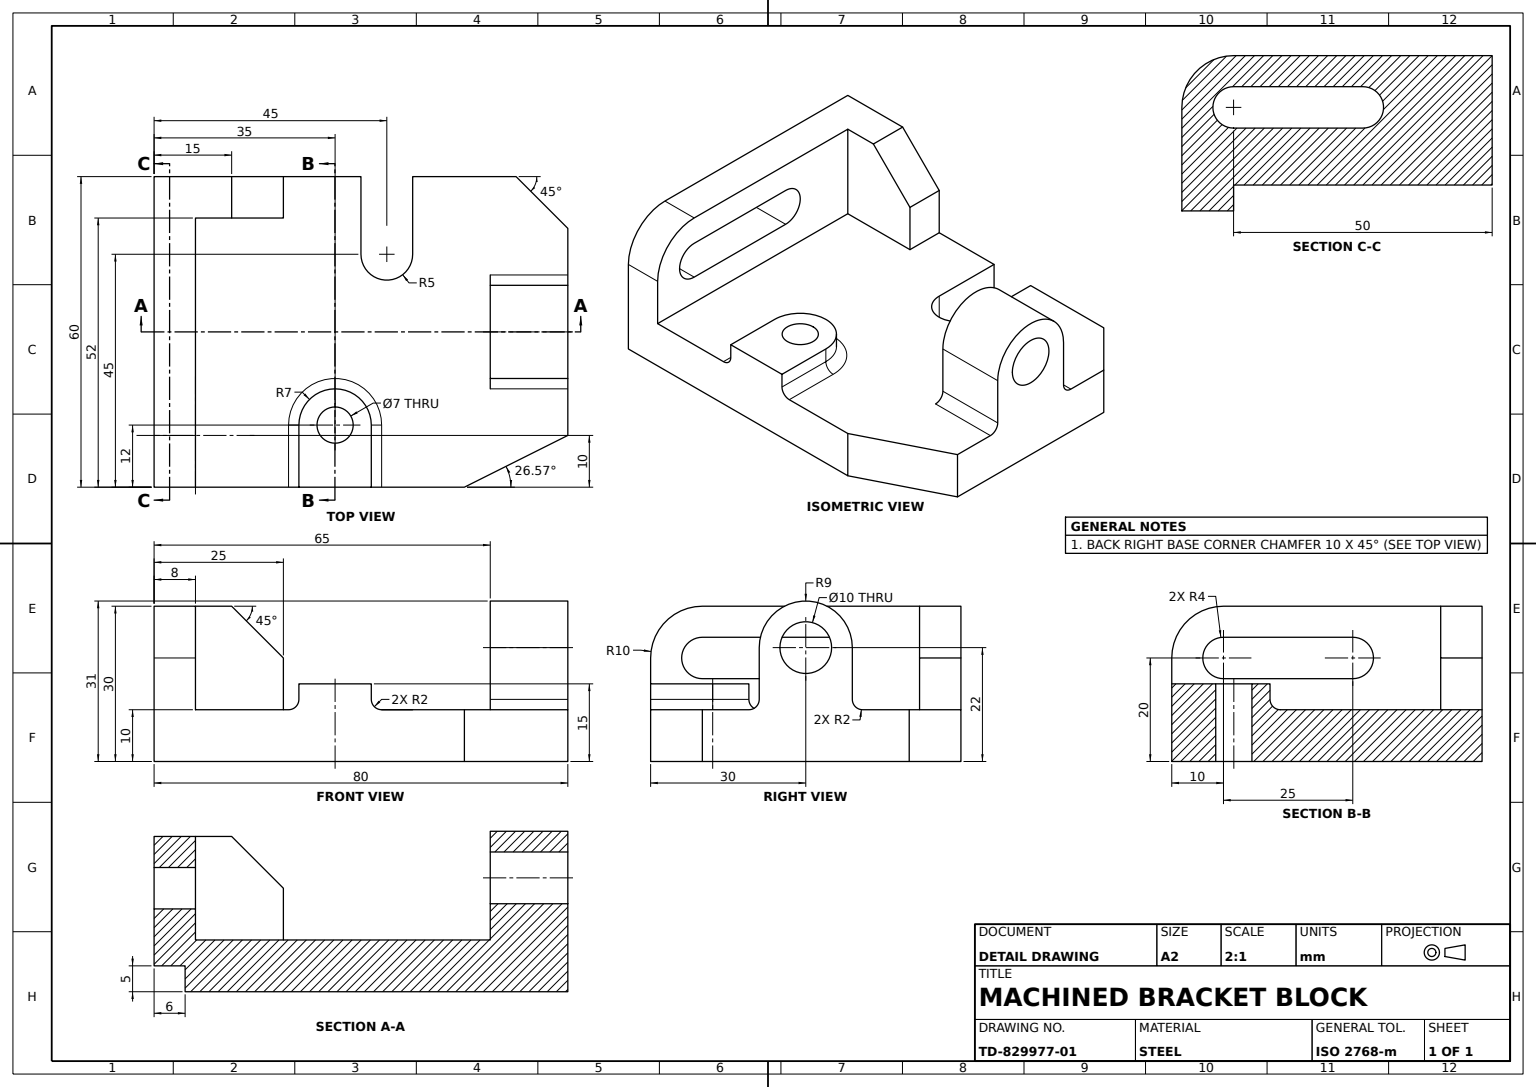
ISO-10303-21;
HEADER;
FILE_DESCRIPTION((''),'2;1');
FILE_NAME('','',(''),(''),'','','');
FILE_SCHEMA(('AUTOMOTIVE_DESIGN'));
ENDSEC;
DATA;
#1=APPLICATION_CONTEXT('');
#2=PRODUCT_CONTEXT('',#1,'mechanical');
#3=PRODUCT('','','',(#2));
#4=PRODUCT_DEFINITION_FORMATION('','',#3);
#5=PRODUCT_DEFINITION_CONTEXT('',#1,'design');
#6=PRODUCT_DEFINITION('','',#4,#5);
#7=PRODUCT_DEFINITION_SHAPE('','',#6);
#8=(LENGTH_UNIT()NAMED_UNIT(*)SI_UNIT(.MILLI.,.METRE.));
#9=(NAMED_UNIT(*)PLANE_ANGLE_UNIT()SI_UNIT($,.RADIAN.));
#10=(NAMED_UNIT(*)SI_UNIT($,.STERADIAN.)SOLID_ANGLE_UNIT());
#11=UNCERTAINTY_MEASURE_WITH_UNIT(LENGTH_MEASURE(1.E-05),#8,'distance_accuracy_value','');
#12=(GEOMETRIC_REPRESENTATION_CONTEXT(3)GLOBAL_UNCERTAINTY_ASSIGNED_CONTEXT((#11))GLOBAL_UNIT_ASSIGNED_CONTEXT((#8,#9,#10))REPRESENTATION_CONTEXT('',''));
#13=CARTESIAN_POINT('',(42.,15.,30.));
#14=VERTEX_POINT('',#13);
#15=CARTESIAN_POINT('',(42.,12.,30.));
#16=VERTEX_POINT('',#15);
#17=DIRECTION('',(0.,-1.,0.));
#18=VECTOR('',#17,1000.);
#19=LINE('',#13,#18);
#20=EDGE_CURVE('',#14,#16,#19,.T.);
#21=ORIENTED_EDGE('',*,*,#20,.T.);
#22=CARTESIAN_POINT('',(42.,12.,18.));
#23=VERTEX_POINT('',#22);
#24=DIRECTION('',(0.,0.,-1.));
#25=VECTOR('',#24,1000.);
#26=LINE('',#15,#25);
#27=EDGE_CURVE('',#16,#23,#26,.T.);
#28=ORIENTED_EDGE('',*,*,#27,.T.);
#29=CARTESIAN_POINT('',(42.,15.,18.));
#30=VERTEX_POINT('',#29);
#31=LINE('',#29,#18);
#32=EDGE_CURVE('',#30,#23,#31,.T.);
#33=ORIENTED_EDGE('',*,*,#32,.F.);
#34=LINE('',#13,#25);
#35=EDGE_CURVE('',#14,#30,#34,.T.);
#36=ORIENTED_EDGE('',*,*,#35,.F.);
#37=EDGE_LOOP('',(#21,#28,#33,#36));
#38=FACE_OUTER_BOUND('',#37,.T.);
#39=DIRECTION('',(-1.,0.,0.));
#40=DIRECTION('',(0.,0.,1.));
#41=AXIS2_PLACEMENT_3D('',#13,#39,#40);
#42=PLANE('',#41);
#43=ADVANCED_FACE('',(#38),#42,.F.);
#44=CARTESIAN_POINT('',(28.,15.,18.));
#45=VERTEX_POINT('',#44);
#46=CARTESIAN_POINT('',(28.,12.,18.));
#47=VERTEX_POINT('',#46);
#48=LINE('',#44,#18);
#49=EDGE_CURVE('',#45,#47,#48,.T.);
#50=ORIENTED_EDGE('',*,*,#49,.F.);
#51=CARTESIAN_POINT('',(35.,15.,11.));
#52=VERTEX_POINT('',#51);
#53=CARTESIAN_POINT('',(35.,15.,18.));
#54=DIRECTION('',(0.,1.,0.));
#55=AXIS2_PLACEMENT_3D('',#53,#54,#40);
#56=CIRCLE('',#55,7.);
#57=EDGE_CURVE('',#52,#45,#56,.T.);
#58=ORIENTED_EDGE('',*,*,#57,.F.);
#59=CARTESIAN_POINT('',(35.,12.,11.));
#60=VERTEX_POINT('',#59);
#61=LINE('',#51,#18);
#62=EDGE_CURVE('',#52,#60,#61,.T.);
#63=ORIENTED_EDGE('',*,*,#62,.T.);
#64=CARTESIAN_POINT('',(35.,12.,18.));
#65=AXIS2_PLACEMENT_3D('',#64,#54,#40);
#66=CIRCLE('',#65,7.);
#67=EDGE_CURVE('',#60,#47,#66,.T.);
#68=ORIENTED_EDGE('',*,*,#67,.T.);
#69=EDGE_LOOP('',(#50,#58,#63,#68));
#70=FACE_OUTER_BOUND('',#69,.T.);
#71=AXIS2_PLACEMENT_3D('',#53,#17,#24);
#72=CYLINDRICAL_SURFACE('',#71,7.);
#73=ADVANCED_FACE('',(#70),#72,.T.);
#74=CARTESIAN_POINT('',(0.,20.,24.));
#75=VERTEX_POINT('',#74);
#76=CARTESIAN_POINT('',(0.,24.,20.));
#77=VERTEX_POINT('',#76);
#78=CARTESIAN_POINT('',(0.,20.,20.));
#79=AXIS2_PLACEMENT_3D('',#78,#39,#40);
#80=CIRCLE('',#79,4.);
#81=EDGE_CURVE('',#75,#77,#80,.T.);
#82=ORIENTED_EDGE('',*,*,#81,.T.);
#83=CARTESIAN_POINT('',(8.,24.,20.));
#84=VERTEX_POINT('',#83);
#85=VECTOR('',#39,1000.);
#86=LINE('',#83,#85);
#87=EDGE_CURVE('',#84,#77,#86,.T.);
#88=ORIENTED_EDGE('',*,*,#87,.F.);
#89=CARTESIAN_POINT('',(8.,20.,24.));
#90=VERTEX_POINT('',#89);
#91=CARTESIAN_POINT('',(8.,20.,20.));
#92=AXIS2_PLACEMENT_3D('',#91,#39,#40);
#93=CIRCLE('',#92,4.);
#94=EDGE_CURVE('',#90,#84,#93,.T.);
#95=ORIENTED_EDGE('',*,*,#94,.F.);
#96=LINE('',#89,#85);
#97=EDGE_CURVE('',#90,#75,#96,.T.);
#98=ORIENTED_EDGE('',*,*,#97,.T.);
#99=EDGE_LOOP('',(#82,#88,#95,#98));
#100=FACE_OUTER_BOUND('',#99,.T.);
#101=CYLINDRICAL_SURFACE('',#92,4.);
#102=ADVANCED_FACE('',(#100),#101,.F.);
#103=CARTESIAN_POINT('',(0.,16.,-5.));
#104=VERTEX_POINT('',#103);
#105=CARTESIAN_POINT('',(0.,16.,20.));
#106=VERTEX_POINT('',#105);
#107=VECTOR('',#40,1000.);
#108=LINE('',#105,#107);
#109=EDGE_CURVE('',#104,#106,#108,.T.);
#110=ORIENTED_EDGE('',*,*,#109,.F.);
#111=CARTESIAN_POINT('',(0.,24.,-5.));
#112=VERTEX_POINT('',#111);
#113=CARTESIAN_POINT('',(0.,20.,-5.));
#114=AXIS2_PLACEMENT_3D('',#113,#39,#40);
#115=CIRCLE('',#114,4.);
#116=EDGE_CURVE('',#112,#104,#115,.T.);
#117=ORIENTED_EDGE('',*,*,#116,.F.);
#118=LINE('',#76,#25);
#119=EDGE_CURVE('',#77,#112,#118,.T.);
#120=ORIENTED_EDGE('',*,*,#119,.F.);
#121=ORIENTED_EDGE('',*,*,#81,.F.);
#122=EDGE_CURVE('',#106,#75,#80,.T.);
#123=ORIENTED_EDGE('',*,*,#122,.F.);
#124=EDGE_LOOP('',(#110,#117,#120,#121,#123));
#125=FACE_BOUND('',#124,.T.);
#126=CARTESIAN_POINT('',(0.,0.,20.));
#127=VERTEX_POINT('',#126);
#128=CARTESIAN_POINT('',(0.,0.,30.));
#129=VERTEX_POINT('',#128);
#130=CARTESIAN_POINT('',(0.,0.,0.));
#131=LINE('',#130,#107);
#132=EDGE_CURVE('',#127,#129,#131,.T.);
#133=ORIENTED_EDGE('',*,*,#132,.T.);
#134=CARTESIAN_POINT('',(0.,20.,30.));
#135=VERTEX_POINT('',#134);
#136=CARTESIAN_POINT('',(0.,10.,30.));
#137=LINE('',#136,#18);
#138=EDGE_CURVE('',#135,#129,#137,.T.);
#139=ORIENTED_EDGE('',*,*,#138,.F.);
#140=CARTESIAN_POINT('',(0.,30.,20.));
#141=VERTEX_POINT('',#140);
#142=CIRCLE('',#79,10.);
#143=EDGE_CURVE('',#135,#141,#142,.T.);
#144=ORIENTED_EDGE('',*,*,#143,.T.);
#145=CARTESIAN_POINT('',(0.,30.,-30.));
#146=VERTEX_POINT('',#145);
#147=LINE('',#140,#25);
#148=EDGE_CURVE('',#141,#146,#147,.T.);
#149=ORIENTED_EDGE('',*,*,#148,.T.);
#150=CARTESIAN_POINT('',(0.,5.,-30.));
#151=VERTEX_POINT('',#150);
#152=CARTESIAN_POINT('',(0.,10.,-30.));
#153=LINE('',#152,#18);
#154=EDGE_CURVE('',#146,#151,#153,.T.);
#155=ORIENTED_EDGE('',*,*,#154,.T.);
#156=CARTESIAN_POINT('',(0.,5.,20.));
#157=VERTEX_POINT('',#156);
#158=LINE('',#156,#25);
#159=EDGE_CURVE('',#157,#151,#158,.T.);
#160=ORIENTED_EDGE('',*,*,#159,.F.);
#161=VECTOR('',#54,1000.);
#162=LINE('',#126,#161);
#163=EDGE_CURVE('',#127,#157,#162,.T.);
#164=ORIENTED_EDGE('',*,*,#163,.F.);
#165=EDGE_LOOP('',(#133,#139,#144,#149,#155,#160,#164));
#166=FACE_OUTER_BOUND('',#165,.T.);
#167=CARTESIAN_POINT('',(0.,10.,0.));
#168=DIRECTION('',(1.,0.,0.));
#169=AXIS2_PLACEMENT_3D('',#167,#168,#24);
#170=PLANE('',#169);
#171=ADVANCED_FACE('',(#125,#166),#170,.F.);
#172=CARTESIAN_POINT('',(8.,16.,-5.));
#173=VERTEX_POINT('',#172);
#174=CARTESIAN_POINT('',(8.,16.,20.));
#175=VERTEX_POINT('',#174);
#176=LINE('',#174,#107);
#177=EDGE_CURVE('',#173,#175,#176,.T.);
#178=ORIENTED_EDGE('',*,*,#177,.F.);
#179=LINE('',#172,#85);
#180=EDGE_CURVE('',#173,#104,#179,.T.);
#181=ORIENTED_EDGE('',*,*,#180,.T.);
#182=ORIENTED_EDGE('',*,*,#109,.T.);
#183=LINE('',#174,#85);
#184=EDGE_CURVE('',#175,#106,#183,.T.);
#185=ORIENTED_EDGE('',*,*,#184,.F.);
#186=EDGE_LOOP('',(#178,#181,#182,#185));
#187=FACE_OUTER_BOUND('',#186,.T.);
#188=AXIS2_PLACEMENT_3D('',#174,#17,#24);
#189=PLANE('',#188);
#190=ADVANCED_FACE('',(#187),#189,.F.);
#191=CARTESIAN_POINT('',(60.,10.,30.));
#192=VERTEX_POINT('',#191);
#193=CARTESIAN_POINT('',(80.,10.,20.));
#194=VERTEX_POINT('',#193);
#195=DIRECTION('',(0.894427191,0.,-0.447213595));
#196=VECTOR('',#195,1000.);
#197=LINE('',#193,#196);
#198=EDGE_CURVE('',#192,#194,#197,.T.);
#199=ORIENTED_EDGE('',*,*,#198,.T.);
#200=CARTESIAN_POINT('',(80.,10.,11.));
#201=VERTEX_POINT('',#200);
#202=CARTESIAN_POINT('',(80.,10.,-30.));
#203=LINE('',#202,#25);
#204=EDGE_CURVE('',#194,#201,#203,.T.);
#205=ORIENTED_EDGE('',*,*,#204,.T.);
#206=CARTESIAN_POINT('',(65.,10.,11.));
#207=VERTEX_POINT('',#206);
#208=LINE('',#206,#85);
#209=EDGE_CURVE('',#201,#207,#208,.T.);
#210=ORIENTED_EDGE('',*,*,#209,.T.);
#211=CARTESIAN_POINT('',(65.,10.,-11.));
#212=VERTEX_POINT('',#211);
#213=CARTESIAN_POINT('',(65.,10.,9.));
#214=LINE('',#213,#25);
#215=EDGE_CURVE('',#207,#212,#214,.T.);
#216=ORIENTED_EDGE('',*,*,#215,.T.);
#217=CARTESIAN_POINT('',(80.,10.,-11.));
#218=VERTEX_POINT('',#217);
#219=VECTOR('',#168,1000.);
#220=LINE('',#217,#219);
#221=EDGE_CURVE('',#212,#218,#220,.T.);
#222=ORIENTED_EDGE('',*,*,#221,.T.);
#223=CARTESIAN_POINT('',(80.,10.,-20.));
#224=VERTEX_POINT('',#223);
#225=EDGE_CURVE('',#218,#224,#203,.T.);
#226=ORIENTED_EDGE('',*,*,#225,.T.);
#227=CARTESIAN_POINT('',(70.,10.,-30.));
#228=VERTEX_POINT('',#227);
#229=CARTESIAN_POINT('',(65.,10.,-35.));
#230=DIRECTION('',(-0.707106781,0.,-0.707106781));
#231=VECTOR('',#230,1000.);
#232=LINE('',#229,#231);
#233=EDGE_CURVE('',#224,#228,#232,.T.);
#234=ORIENTED_EDGE('',*,*,#233,.T.);
#235=CARTESIAN_POINT('',(50.,10.,-30.));
#236=VERTEX_POINT('',#235);
#237=LINE('',#235,#85);
#238=EDGE_CURVE('',#228,#236,#237,.T.);
#239=ORIENTED_EDGE('',*,*,#238,.T.);
#240=CARTESIAN_POINT('',(50.,10.,-15.));
#241=VERTEX_POINT('',#240);
#242=LINE('',#240,#107);
#243=EDGE_CURVE('',#236,#241,#242,.T.);
#244=ORIENTED_EDGE('',*,*,#243,.T.);
#245=CARTESIAN_POINT('',(40.,10.,-15.));
#246=VERTEX_POINT('',#245);
#247=CARTESIAN_POINT('',(45.,10.,-15.));
#248=AXIS2_PLACEMENT_3D('',#247,#17,#40);
#249=CIRCLE('',#248,5.);
#250=EDGE_CURVE('',#241,#246,#249,.T.);
#251=ORIENTED_EDGE('',*,*,#250,.T.);
#252=CARTESIAN_POINT('',(40.,10.,-30.));
#253=VERTEX_POINT('',#252);
#254=LINE('',#252,#25);
#255=EDGE_CURVE('',#246,#253,#254,.T.);
#256=ORIENTED_EDGE('',*,*,#255,.T.);
#257=CARTESIAN_POINT('',(25.,10.,-30.));
#258=VERTEX_POINT('',#257);
#259=LINE('',#152,#85);
#260=EDGE_CURVE('',#253,#258,#259,.T.);
#261=ORIENTED_EDGE('',*,*,#260,.T.);
#262=CARTESIAN_POINT('',(25.,10.,-22.));
#263=VERTEX_POINT('',#262);
#264=LINE('',#262,#25);
#265=EDGE_CURVE('',#263,#258,#264,.T.);
#266=ORIENTED_EDGE('',*,*,#265,.F.);
#267=CARTESIAN_POINT('',(8.,10.,-22.));
#268=VERTEX_POINT('',#267);
#269=LINE('',#262,#85);
#270=EDGE_CURVE('',#263,#268,#269,.T.);
#271=ORIENTED_EDGE('',*,*,#270,.T.);
#272=CARTESIAN_POINT('',(8.,10.,30.));
#273=VERTEX_POINT('',#272);
#274=CARTESIAN_POINT('',(8.,10.,-30.));
#275=LINE('',#274,#107);
#276=EDGE_CURVE('',#268,#273,#275,.T.);
#277=ORIENTED_EDGE('',*,*,#276,.T.);
#278=CARTESIAN_POINT('',(26.,10.,30.));
#279=VERTEX_POINT('',#278);
#280=LINE('',#191,#219);
#281=EDGE_CURVE('',#273,#279,#280,.T.);
#282=ORIENTED_EDGE('',*,*,#281,.T.);
#283=CARTESIAN_POINT('',(26.,10.,18.));
#284=VERTEX_POINT('',#283);
#285=CARTESIAN_POINT('',(26.,10.,-15.));
#286=LINE('',#285,#25);
#287=EDGE_CURVE('',#279,#284,#286,.T.);
#288=ORIENTED_EDGE('',*,*,#287,.T.);
#289=CARTESIAN_POINT('',(44.,10.,18.));
#290=VERTEX_POINT('',#289);
#291=CARTESIAN_POINT('',(35.,10.,18.));
#292=AXIS2_PLACEMENT_3D('',#291,#17,#40);
#293=CIRCLE('',#292,9.);
#294=EDGE_CURVE('',#284,#290,#293,.T.);
#295=ORIENTED_EDGE('',*,*,#294,.T.);
#296=CARTESIAN_POINT('',(44.,10.,30.));
#297=VERTEX_POINT('',#296);
#298=CARTESIAN_POINT('',(44.,10.,-15.));
#299=LINE('',#298,#107);
#300=EDGE_CURVE('',#290,#297,#299,.T.);
#301=ORIENTED_EDGE('',*,*,#300,.T.);
#302=EDGE_CURVE('',#297,#192,#280,.T.);
#303=ORIENTED_EDGE('',*,*,#302,.T.);
#304=EDGE_LOOP('',(#199,#205,#210,#216,#222,#226,#234,#239,#244,#251,#256,#261,#266,#271,#277,#282,#288,#295,#301,#303));
#305=FACE_OUTER_BOUND('',#304,.T.);
#306=AXIS2_PLACEMENT_3D('',#247,#54,#40);
#307=PLANE('',#306);
#308=ADVANCED_FACE('',(#305),#307,.T.);
#309=ORIENTED_EDGE('',*,*,#184,.T.);
#310=ORIENTED_EDGE('',*,*,#122,.T.);
#311=ORIENTED_EDGE('',*,*,#97,.F.);
#312=EDGE_CURVE('',#175,#90,#93,.T.);
#313=ORIENTED_EDGE('',*,*,#312,.F.);
#314=EDGE_LOOP('',(#309,#310,#311,#313));
#315=FACE_OUTER_BOUND('',#314,.T.);
#316=ADVANCED_FACE('',(#315),#101,.F.);
#317=CARTESIAN_POINT('',(8.,20.,30.));
#318=VERTEX_POINT('',#317);
#319=LINE('',#317,#85);
#320=EDGE_CURVE('',#318,#135,#319,.T.);
#321=ORIENTED_EDGE('',*,*,#320,.F.);
#322=CARTESIAN_POINT('',(8.,30.,20.));
#323=VERTEX_POINT('',#322);
#324=CIRCLE('',#92,10.);
#325=EDGE_CURVE('',#318,#323,#324,.T.);
#326=ORIENTED_EDGE('',*,*,#325,.T.);
#327=LINE('',#322,#85);
#328=EDGE_CURVE('',#323,#141,#327,.T.);
#329=ORIENTED_EDGE('',*,*,#328,.T.);
#330=ORIENTED_EDGE('',*,*,#143,.F.);
#331=EDGE_LOOP('',(#321,#326,#329,#330));
#332=FACE_OUTER_BOUND('',#331,.T.);
#333=CYLINDRICAL_SURFACE('',#92,10.);
#334=ADVANCED_FACE('',(#332),#333,.T.);
#335=CARTESIAN_POINT('',(28.,12.,30.));
#336=VERTEX_POINT('',#335);
#337=CARTESIAN_POINT('',(26.,12.,30.));
#338=AXIS2_PLACEMENT_3D('',#337,#24,#39);
#339=CIRCLE('',#338,2.);
#340=EDGE_CURVE('',#336,#279,#339,.T.);
#341=ORIENTED_EDGE('',*,*,#340,.T.);
#342=ORIENTED_EDGE('',*,*,#281,.F.);
#343=LINE('',#317,#161);
#344=EDGE_CURVE('',#273,#318,#343,.T.);
#345=ORIENTED_EDGE('',*,*,#344,.T.);
#346=ORIENTED_EDGE('',*,*,#320,.T.);
#347=ORIENTED_EDGE('',*,*,#138,.T.);
#348=CARTESIAN_POINT('',(60.,0.,30.));
#349=VERTEX_POINT('',#348);
#350=LINE('',#348,#219);
#351=EDGE_CURVE('',#129,#349,#350,.T.);
#352=ORIENTED_EDGE('',*,*,#351,.T.);
#353=LINE('',#191,#18);
#354=EDGE_CURVE('',#192,#349,#353,.T.);
#355=ORIENTED_EDGE('',*,*,#354,.F.);
#356=ORIENTED_EDGE('',*,*,#302,.F.);
#357=CARTESIAN_POINT('',(44.,12.,30.));
#358=AXIS2_PLACEMENT_3D('',#357,#24,#39);
#359=CIRCLE('',#358,2.);
#360=EDGE_CURVE('',#297,#16,#359,.T.);
#361=ORIENTED_EDGE('',*,*,#360,.T.);
#362=ORIENTED_EDGE('',*,*,#20,.F.);
#363=CARTESIAN_POINT('',(28.,15.,30.));
#364=VERTEX_POINT('',#363);
#365=LINE('',#363,#219);
#366=EDGE_CURVE('',#364,#14,#365,.T.);
#367=ORIENTED_EDGE('',*,*,#366,.F.);
#368=LINE('',#363,#18);
#369=EDGE_CURVE('',#364,#336,#368,.T.);
#370=ORIENTED_EDGE('',*,*,#369,.T.);
#371=EDGE_LOOP('',(#341,#342,#345,#346,#347,#352,#355,#356,#361,#362,#367,#370));
#372=FACE_OUTER_BOUND('',#371,.T.);
#373=AXIS2_PLACEMENT_3D('',#191,#24,#39);
#374=PLANE('',#373);
#375=ADVANCED_FACE('',(#372),#374,.F.);
#376=ORIENTED_EDGE('',*,*,#119,.T.);
#377=CARTESIAN_POINT('',(8.,24.,-5.));
#378=VERTEX_POINT('',#377);
#379=LINE('',#377,#85);
#380=EDGE_CURVE('',#378,#112,#379,.T.);
#381=ORIENTED_EDGE('',*,*,#380,.F.);
#382=LINE('',#83,#25);
#383=EDGE_CURVE('',#84,#378,#382,.T.);
#384=ORIENTED_EDGE('',*,*,#383,.F.);
#385=ORIENTED_EDGE('',*,*,#87,.T.);
#386=EDGE_LOOP('',(#376,#381,#384,#385));
#387=FACE_OUTER_BOUND('',#386,.T.);
#388=AXIS2_PLACEMENT_3D('',#83,#54,#40);
#389=PLANE('',#388);
#390=ADVANCED_FACE('',(#387),#389,.F.);
#391=CARTESIAN_POINT('',(80.,22.,5.));
#392=VERTEX_POINT('',#391);
#393=CARTESIAN_POINT('',(80.,22.,-5.));
#394=VERTEX_POINT('',#393);
#395=CARTESIAN_POINT('',(80.,22.,0.));
#396=AXIS2_PLACEMENT_3D('',#395,#168,#24);
#397=CIRCLE('',#396,5.);
#398=EDGE_CURVE('',#392,#394,#397,.T.);
#399=ORIENTED_EDGE('',*,*,#398,.F.);
#400=EDGE_CURVE('',#394,#392,#397,.T.);
#401=ORIENTED_EDGE('',*,*,#400,.F.);
#402=EDGE_LOOP('',(#399,#401));
#403=FACE_BOUND('',#402,.T.);
#404=CARTESIAN_POINT('',(80.,12.,-9.));
#405=VERTEX_POINT('',#404);
#406=CARTESIAN_POINT('',(80.,12.,-11.));
#407=AXIS2_PLACEMENT_3D('',#406,#39,#40);
#408=CIRCLE('',#407,2.);
#409=EDGE_CURVE('',#218,#405,#408,.T.);
#410=ORIENTED_EDGE('',*,*,#409,.T.);
#411=CARTESIAN_POINT('',(80.,22.,-9.));
#412=VERTEX_POINT('',#411);
#413=CARTESIAN_POINT('',(80.,10.,-9.));
#414=LINE('',#413,#161);
#415=EDGE_CURVE('',#405,#412,#414,.T.);
#416=ORIENTED_EDGE('',*,*,#415,.T.);
#417=CARTESIAN_POINT('',(80.,22.,9.));
#418=VERTEX_POINT('',#417);
#419=CIRCLE('',#396,9.);
#420=EDGE_CURVE('',#412,#418,#419,.T.);
#421=ORIENTED_EDGE('',*,*,#420,.T.);
#422=CARTESIAN_POINT('',(80.,12.,9.));
#423=VERTEX_POINT('',#422);
#424=LINE('',#417,#18);
#425=EDGE_CURVE('',#418,#423,#424,.T.);
#426=ORIENTED_EDGE('',*,*,#425,.T.);
#427=CARTESIAN_POINT('',(80.,12.,11.));
#428=AXIS2_PLACEMENT_3D('',#427,#39,#40);
#429=CIRCLE('',#428,2.);
#430=EDGE_CURVE('',#423,#201,#429,.T.);
#431=ORIENTED_EDGE('',*,*,#430,.T.);
#432=ORIENTED_EDGE('',*,*,#204,.F.);
#433=CARTESIAN_POINT('',(80.,0.,20.));
#434=VERTEX_POINT('',#433);
#435=LINE('',#193,#18);
#436=EDGE_CURVE('',#194,#434,#435,.T.);
#437=ORIENTED_EDGE('',*,*,#436,.T.);
#438=CARTESIAN_POINT('',(80.,0.,-20.));
#439=VERTEX_POINT('',#438);
#440=CARTESIAN_POINT('',(80.,0.,-30.));
#441=LINE('',#440,#25);
#442=EDGE_CURVE('',#434,#439,#441,.T.);
#443=ORIENTED_EDGE('',*,*,#442,.T.);
#444=LINE('',#223,#161);
#445=EDGE_CURVE('',#439,#224,#444,.T.);
#446=ORIENTED_EDGE('',*,*,#445,.T.);
#447=ORIENTED_EDGE('',*,*,#225,.F.);
#448=EDGE_LOOP('',(#410,#416,#421,#426,#431,#432,#437,#443,#446,#447));
#449=FACE_OUTER_BOUND('',#448,.T.);
#450=AXIS2_PLACEMENT_3D('',#202,#39,#40);
#451=PLANE('',#450);
#452=ADVANCED_FACE('',(#403,#449),#451,.F.);
#453=CARTESIAN_POINT('',(40.,0.,-15.));
#454=VERTEX_POINT('',#453);
#455=LINE('',#245,#18);
#456=EDGE_CURVE('',#246,#454,#455,.T.);
#457=ORIENTED_EDGE('',*,*,#456,.F.);
#458=ORIENTED_EDGE('',*,*,#250,.F.);
#459=CARTESIAN_POINT('',(50.,0.,-15.));
#460=VERTEX_POINT('',#459);
#461=LINE('',#240,#18);
#462=EDGE_CURVE('',#241,#460,#461,.T.);
#463=ORIENTED_EDGE('',*,*,#462,.T.);
#464=CARTESIAN_POINT('',(45.,0.,-15.));
#465=AXIS2_PLACEMENT_3D('',#464,#17,#40);
#466=CIRCLE('',#465,5.);
#467=EDGE_CURVE('',#460,#454,#466,.T.);
#468=ORIENTED_EDGE('',*,*,#467,.T.);
#469=EDGE_LOOP('',(#457,#458,#463,#468));
#470=FACE_OUTER_BOUND('',#469,.T.);
#471=AXIS2_PLACEMENT_3D('',#247,#17,#24);
#472=CYLINDRICAL_SURFACE('',#471,5.);
#473=ADVANCED_FACE('',(#470),#472,.F.);
#474=ORIENTED_EDGE('',*,*,#154,.F.);
#475=CARTESIAN_POINT('',(15.,30.,-30.));
#476=VERTEX_POINT('',#475);
#477=CARTESIAN_POINT('',(8.,30.,-30.));
#478=LINE('',#477,#85);
#479=EDGE_CURVE('',#476,#146,#478,.T.);
#480=ORIENTED_EDGE('',*,*,#479,.F.);
#481=CARTESIAN_POINT('',(25.,20.,-30.));
#482=VERTEX_POINT('',#481);
#483=DIRECTION('',(0.707106781,-0.707106781,0.));
#484=VECTOR('',#483,1000.);
#485=LINE('',#475,#484);
#486=EDGE_CURVE('',#476,#482,#485,.T.);
#487=ORIENTED_EDGE('',*,*,#486,.T.);
#488=CARTESIAN_POINT('',(25.,30.,-30.));
#489=LINE('',#488,#18);
#490=EDGE_CURVE('',#482,#258,#489,.T.);
#491=ORIENTED_EDGE('',*,*,#490,.T.);
#492=ORIENTED_EDGE('',*,*,#260,.F.);
#493=CARTESIAN_POINT('',(40.,0.,-30.));
#494=VERTEX_POINT('',#493);
#495=LINE('',#252,#18);
#496=EDGE_CURVE('',#253,#494,#495,.T.);
#497=ORIENTED_EDGE('',*,*,#496,.T.);
#498=CARTESIAN_POINT('',(6.,0.,-30.));
#499=VERTEX_POINT('',#498);
#500=CARTESIAN_POINT('',(0.,0.,-30.));
#501=LINE('',#500,#85);
#502=EDGE_CURVE('',#494,#499,#501,.T.);
#503=ORIENTED_EDGE('',*,*,#502,.T.);
#504=CARTESIAN_POINT('',(6.,5.,-30.));
#505=VERTEX_POINT('',#504);
#506=LINE('',#498,#18);
#507=EDGE_CURVE('',#505,#499,#506,.T.);
#508=ORIENTED_EDGE('',*,*,#507,.F.);
#509=LINE('',#150,#219);
#510=EDGE_CURVE('',#151,#505,#509,.T.);
#511=ORIENTED_EDGE('',*,*,#510,.F.);
#512=EDGE_LOOP('',(#474,#480,#487,#491,#492,#497,#503,#508,#511));
#513=FACE_OUTER_BOUND('',#512,.T.);
#514=AXIS2_PLACEMENT_3D('',#152,#40,#168);
#515=PLANE('',#514);
#516=ADVANCED_FACE('',(#513),#515,.F.);
#517=CARTESIAN_POINT('',(35.,0.,21.5));
#518=VERTEX_POINT('',#517);
#519=CARTESIAN_POINT('',(35.,0.,14.5));
#520=VERTEX_POINT('',#519);
#521=CARTESIAN_POINT('',(35.,0.,18.));
#522=AXIS2_PLACEMENT_3D('',#521,#54,#40);
#523=CIRCLE('',#522,3.5);
#524=EDGE_CURVE('',#518,#520,#523,.T.);
#525=ORIENTED_EDGE('',*,*,#524,.F.);
#526=CARTESIAN_POINT('',(35.,15.,21.5));
#527=VERTEX_POINT('',#526);
#528=LINE('',#517,#161);
#529=EDGE_CURVE('',#518,#527,#528,.T.);
#530=ORIENTED_EDGE('',*,*,#529,.T.);
#531=CARTESIAN_POINT('',(35.,15.,14.5));
#532=VERTEX_POINT('',#531);
#533=CIRCLE('',#55,3.5);
#534=EDGE_CURVE('',#527,#532,#533,.T.);
#535=ORIENTED_EDGE('',*,*,#534,.T.);
#536=LINE('',#519,#161);
#537=EDGE_CURVE('',#520,#532,#536,.T.);
#538=ORIENTED_EDGE('',*,*,#537,.F.);
#539=EDGE_LOOP('',(#525,#530,#535,#538));
#540=FACE_OUTER_BOUND('',#539,.T.);
#541=CYLINDRICAL_SURFACE('',#522,3.5);
#542=ADVANCED_FACE('',(#540),#541,.F.);
#543=CARTESIAN_POINT('',(65.,12.,9.));
#544=VERTEX_POINT('',#543);
#545=CARTESIAN_POINT('',(65.,12.,11.));
#546=AXIS2_PLACEMENT_3D('',#545,#168,#24);
#547=CIRCLE('',#546,2.);
#548=EDGE_CURVE('',#207,#544,#547,.T.);
#549=ORIENTED_EDGE('',*,*,#548,.F.);
#550=ORIENTED_EDGE('',*,*,#209,.F.);
#551=ORIENTED_EDGE('',*,*,#430,.F.);
#552=LINE('',#422,#219);
#553=EDGE_CURVE('',#544,#423,#552,.T.);
#554=ORIENTED_EDGE('',*,*,#553,.F.);
#555=EDGE_LOOP('',(#549,#550,#551,#554));
#556=FACE_OUTER_BOUND('',#555,.T.);
#557=AXIS2_PLACEMENT_3D('',#545,#39,#40);
#558=CYLINDRICAL_SURFACE('',#557,2.);
#559=ADVANCED_FACE('',(#556),#558,.F.);
#560=CARTESIAN_POINT('',(26.,12.,18.));
#561=AXIS2_PLACEMENT_3D('',#560,#24,#39);
#562=CIRCLE('',#561,2.);
#563=EDGE_CURVE('',#47,#284,#562,.T.);
#564=ORIENTED_EDGE('',*,*,#563,.T.);
#565=ORIENTED_EDGE('',*,*,#287,.F.);
#566=ORIENTED_EDGE('',*,*,#340,.F.);
#567=LINE('',#46,#107);
#568=EDGE_CURVE('',#47,#336,#567,.T.);
#569=ORIENTED_EDGE('',*,*,#568,.F.);
#570=EDGE_LOOP('',(#564,#565,#566,#569));
#571=FACE_OUTER_BOUND('',#570,.T.);
#572=AXIS2_PLACEMENT_3D('',#560,#40,#168);
#573=CYLINDRICAL_SURFACE('',#572,2.);
#574=ADVANCED_FACE('',(#571),#573,.F.);
#575=ORIENTED_EDGE('',*,*,#163,.T.);
#576=CARTESIAN_POINT('',(6.,5.,20.));
#577=VERTEX_POINT('',#576);
#578=LINE('',#156,#219);
#579=EDGE_CURVE('',#157,#577,#578,.T.);
#580=ORIENTED_EDGE('',*,*,#579,.T.);
#581=CARTESIAN_POINT('',(6.,0.,20.));
#582=VERTEX_POINT('',#581);
#583=LINE('',#581,#18);
#584=EDGE_CURVE('',#577,#582,#583,.T.);
#585=ORIENTED_EDGE('',*,*,#584,.T.);
#586=LINE('',#126,#85);
#587=EDGE_CURVE('',#582,#127,#586,.T.);
#588=ORIENTED_EDGE('',*,*,#587,.T.);
#589=EDGE_LOOP('',(#575,#580,#585,#588));
#590=FACE_OUTER_BOUND('',#589,.T.);
#591=AXIS2_PLACEMENT_3D('',#126,#24,#39);
#592=PLANE('',#591);
#593=ADVANCED_FACE('',(#590),#592,.T.);
#594=CARTESIAN_POINT('',(65.,22.,-5.));
#595=VERTEX_POINT('',#594);
#596=CARTESIAN_POINT('',(65.,22.,5.));
#597=VERTEX_POINT('',#596);
#598=CARTESIAN_POINT('',(65.,22.,0.));
#599=AXIS2_PLACEMENT_3D('',#598,#168,#24);
#600=CIRCLE('',#599,5.);
#601=EDGE_CURVE('',#595,#597,#600,.T.);
#602=ORIENTED_EDGE('',*,*,#601,.T.);
#603=EDGE_CURVE('',#597,#595,#600,.T.);
#604=ORIENTED_EDGE('',*,*,#603,.T.);
#605=EDGE_LOOP('',(#602,#604));
#606=FACE_BOUND('',#605,.T.);
#607=ORIENTED_EDGE('',*,*,#548,.T.);
#608=CARTESIAN_POINT('',(65.,22.,9.));
#609=VERTEX_POINT('',#608);
#610=LINE('',#608,#18);
#611=EDGE_CURVE('',#609,#544,#610,.T.);
#612=ORIENTED_EDGE('',*,*,#611,.F.);
#613=CARTESIAN_POINT('',(65.,22.,-9.));
#614=VERTEX_POINT('',#613);
#615=CIRCLE('',#599,9.);
#616=EDGE_CURVE('',#614,#609,#615,.T.);
#617=ORIENTED_EDGE('',*,*,#616,.F.);
#618=CARTESIAN_POINT('',(65.,12.,-9.));
#619=VERTEX_POINT('',#618);
#620=CARTESIAN_POINT('',(65.,10.,-9.));
#621=LINE('',#620,#161);
#622=EDGE_CURVE('',#619,#614,#621,.T.);
#623=ORIENTED_EDGE('',*,*,#622,.F.);
#624=CARTESIAN_POINT('',(65.,12.,-11.));
#625=AXIS2_PLACEMENT_3D('',#624,#168,#24);
#626=CIRCLE('',#625,2.);
#627=EDGE_CURVE('',#619,#212,#626,.T.);
#628=ORIENTED_EDGE('',*,*,#627,.T.);
#629=ORIENTED_EDGE('',*,*,#215,.F.);
#630=EDGE_LOOP('',(#607,#612,#617,#623,#628,#629));
#631=FACE_OUTER_BOUND('',#630,.T.);
#632=PLANE('',#599);
#633=ADVANCED_FACE('',(#606,#631),#632,.F.);
#634=ORIENTED_EDGE('',*,*,#62,.F.);
#635=EDGE_CURVE('',#30,#52,#56,.T.);
#636=ORIENTED_EDGE('',*,*,#635,.F.);
#637=ORIENTED_EDGE('',*,*,#32,.T.);
#638=EDGE_CURVE('',#23,#60,#66,.T.);
#639=ORIENTED_EDGE('',*,*,#638,.T.);
#640=EDGE_LOOP('',(#634,#636,#637,#639));
#641=FACE_OUTER_BOUND('',#640,.T.);
#642=ADVANCED_FACE('',(#641),#72,.T.);
#643=ORIENTED_EDGE('',*,*,#243,.F.);
#644=CARTESIAN_POINT('',(50.,0.,-30.));
#645=VERTEX_POINT('',#644);
#646=LINE('',#235,#18);
#647=EDGE_CURVE('',#236,#645,#646,.T.);
#648=ORIENTED_EDGE('',*,*,#647,.T.);
#649=LINE('',#459,#107);
#650=EDGE_CURVE('',#645,#460,#649,.T.);
#651=ORIENTED_EDGE('',*,*,#650,.T.);
#652=ORIENTED_EDGE('',*,*,#462,.F.);
#653=EDGE_LOOP('',(#643,#648,#651,#652));
#654=FACE_OUTER_BOUND('',#653,.T.);
#655=AXIS2_PLACEMENT_3D('',#240,#168,#24);
#656=PLANE('',#655);
#657=ADVANCED_FACE('',(#654),#656,.F.);
#658=ORIENTED_EDGE('',*,*,#584,.F.);
#659=LINE('',#576,#25);
#660=EDGE_CURVE('',#577,#505,#659,.T.);
#661=ORIENTED_EDGE('',*,*,#660,.T.);
#662=ORIENTED_EDGE('',*,*,#507,.T.);
#663=LINE('',#581,#25);
#664=EDGE_CURVE('',#582,#499,#663,.T.);
#665=ORIENTED_EDGE('',*,*,#664,.F.);
#666=EDGE_LOOP('',(#658,#661,#662,#665));
#667=FACE_OUTER_BOUND('',#666,.T.);
#668=AXIS2_PLACEMENT_3D('',#581,#168,#24);
#669=PLANE('',#668);
#670=ADVANCED_FACE('',(#667),#669,.F.);
#671=ORIENTED_EDGE('',*,*,#328,.F.);
#672=CARTESIAN_POINT('',(8.,30.,-22.));
#673=VERTEX_POINT('',#672);
#674=LINE('',#322,#25);
#675=EDGE_CURVE('',#323,#673,#674,.T.);
#676=ORIENTED_EDGE('',*,*,#675,.T.);
#677=CARTESIAN_POINT('',(15.,30.,-22.));
#678=VERTEX_POINT('',#677);
#679=LINE('',#672,#219);
#680=EDGE_CURVE('',#673,#678,#679,.T.);
#681=ORIENTED_EDGE('',*,*,#680,.T.);
#682=CARTESIAN_POINT('',(15.,30.,20.));
#683=LINE('',#682,#25);
#684=EDGE_CURVE('',#678,#476,#683,.T.);
#685=ORIENTED_EDGE('',*,*,#684,.T.);
#686=ORIENTED_EDGE('',*,*,#479,.T.);
#687=ORIENTED_EDGE('',*,*,#148,.F.);
#688=EDGE_LOOP('',(#671,#676,#681,#685,#686,#687));
#689=FACE_OUTER_BOUND('',#688,.T.);
#690=AXIS2_PLACEMENT_3D('',#322,#54,#40);
#691=PLANE('',#690);
#692=ADVANCED_FACE('',(#689),#691,.T.);
#693=ORIENTED_EDGE('',*,*,#180,.F.);
#694=CARTESIAN_POINT('',(8.,20.,-5.));
#695=AXIS2_PLACEMENT_3D('',#694,#39,#40);
#696=CIRCLE('',#695,4.);
#697=EDGE_CURVE('',#378,#173,#696,.T.);
#698=ORIENTED_EDGE('',*,*,#697,.F.);
#699=ORIENTED_EDGE('',*,*,#380,.T.);
#700=ORIENTED_EDGE('',*,*,#116,.T.);
#701=EDGE_LOOP('',(#693,#698,#699,#700));
#702=FACE_OUTER_BOUND('',#701,.T.);
#703=CYLINDRICAL_SURFACE('',#695,4.);
#704=ADVANCED_FACE('',(#702),#703,.F.);
#705=LINE('',#596,#219);
#706=EDGE_CURVE('',#597,#392,#705,.T.);
#707=ORIENTED_EDGE('',*,*,#706,.F.);
#708=ORIENTED_EDGE('',*,*,#601,.F.);
#709=LINE('',#594,#219);
#710=EDGE_CURVE('',#595,#394,#709,.T.);
#711=ORIENTED_EDGE('',*,*,#710,.T.);
#712=ORIENTED_EDGE('',*,*,#400,.T.);
#713=EDGE_LOOP('',(#707,#708,#711,#712));
#714=FACE_OUTER_BOUND('',#713,.T.);
#715=CYLINDRICAL_SURFACE('',#599,5.);
#716=ADVANCED_FACE('',(#714),#715,.F.);
#717=EDGE_CURVE('',#520,#518,#523,.T.);
#718=ORIENTED_EDGE('',*,*,#717,.T.);
#719=ORIENTED_EDGE('',*,*,#524,.T.);
#720=EDGE_LOOP('',(#718,#719));
#721=FACE_BOUND('',#720,.T.);
#722=CARTESIAN_POINT('',(70.,0.,-30.));
#723=VERTEX_POINT('',#722);
#724=DIRECTION('',(0.707106781,0.,0.707106781));
#725=VECTOR('',#724,1000.);
#726=LINE('',#722,#725);
#727=EDGE_CURVE('',#723,#439,#726,.T.);
#728=ORIENTED_EDGE('',*,*,#727,.T.);
#729=ORIENTED_EDGE('',*,*,#442,.F.);
#730=LINE('',#433,#196);
#731=EDGE_CURVE('',#349,#434,#730,.T.);
#732=ORIENTED_EDGE('',*,*,#731,.F.);
#733=ORIENTED_EDGE('',*,*,#351,.F.);
#734=ORIENTED_EDGE('',*,*,#132,.F.);
#735=ORIENTED_EDGE('',*,*,#587,.F.);
#736=ORIENTED_EDGE('',*,*,#664,.T.);
#737=ORIENTED_EDGE('',*,*,#502,.F.);
#738=LINE('',#493,#25);
#739=EDGE_CURVE('',#454,#494,#738,.T.);
#740=ORIENTED_EDGE('',*,*,#739,.F.);
#741=ORIENTED_EDGE('',*,*,#467,.F.);
#742=ORIENTED_EDGE('',*,*,#650,.F.);
#743=LINE('',#644,#85);
#744=EDGE_CURVE('',#723,#645,#743,.T.);
#745=ORIENTED_EDGE('',*,*,#744,.F.);
#746=EDGE_LOOP('',(#728,#729,#732,#733,#734,#735,#736,#737,#740,#741,#742,#745));
#747=FACE_OUTER_BOUND('',#746,.T.);
#748=AXIS2_PLACEMENT_3D('',#464,#54,#40);
#749=PLANE('',#748);
#750=ADVANCED_FACE('',(#721,#747),#749,.F.);
#751=ORIENTED_EDGE('',*,*,#563,.F.);
#752=ORIENTED_EDGE('',*,*,#67,.F.);
#753=ORIENTED_EDGE('',*,*,#638,.F.);
#754=CARTESIAN_POINT('',(44.,12.,18.));
#755=AXIS2_PLACEMENT_3D('',#754,#40,#168);
#756=CIRCLE('',#755,2.);
#757=EDGE_CURVE('',#23,#290,#756,.T.);
#758=ORIENTED_EDGE('',*,*,#757,.T.);
#759=ORIENTED_EDGE('',*,*,#294,.F.);
#760=EDGE_LOOP('',(#751,#752,#753,#758,#759));
#761=FACE_OUTER_BOUND('',#760,.T.);
#762=TOROIDAL_SURFACE('',#65,9.,2.);
#763=ADVANCED_FACE('',(#761),#762,.F.);
#764=ORIENTED_EDGE('',*,*,#486,.F.);
#765=ORIENTED_EDGE('',*,*,#684,.F.);
#766=CARTESIAN_POINT('',(25.,20.,-22.));
#767=VERTEX_POINT('',#766);
#768=DIRECTION('',(-0.707106781,0.707106781,0.));
#769=VECTOR('',#768,1000.);
#770=LINE('',#677,#769);
#771=EDGE_CURVE('',#767,#678,#770,.T.);
#772=ORIENTED_EDGE('',*,*,#771,.F.);
#773=LINE('',#766,#107);
#774=EDGE_CURVE('',#482,#767,#773,.T.);
#775=ORIENTED_EDGE('',*,*,#774,.F.);
#776=EDGE_LOOP('',(#764,#765,#772,#775));
#777=FACE_OUTER_BOUND('',#776,.T.);
#778=DIRECTION('',(-0.707106781,-0.707106781,0.));
#779=AXIS2_PLACEMENT_3D('',#682,#778,#24);
#780=PLANE('',#779);
#781=ADVANCED_FACE('',(#777),#780,.F.);
#782=ORIENTED_EDGE('',*,*,#369,.F.);
#783=LINE('',#44,#107);
#784=EDGE_CURVE('',#45,#364,#783,.T.);
#785=ORIENTED_EDGE('',*,*,#784,.F.);
#786=ORIENTED_EDGE('',*,*,#49,.T.);
#787=ORIENTED_EDGE('',*,*,#568,.T.);
#788=EDGE_LOOP('',(#782,#785,#786,#787));
#789=FACE_OUTER_BOUND('',#788,.T.);
#790=AXIS2_PLACEMENT_3D('',#44,#168,#24);
#791=PLANE('',#790);
#792=ADVANCED_FACE('',(#789),#791,.F.);
#793=LINE('',#267,#161);
#794=EDGE_CURVE('',#268,#673,#793,.T.);
#795=ORIENTED_EDGE('',*,*,#794,.F.);
#796=ORIENTED_EDGE('',*,*,#270,.F.);
#797=CARTESIAN_POINT('',(25.,30.,-22.));
#798=LINE('',#797,#18);
#799=EDGE_CURVE('',#767,#263,#798,.T.);
#800=ORIENTED_EDGE('',*,*,#799,.F.);
#801=ORIENTED_EDGE('',*,*,#771,.T.);
#802=ORIENTED_EDGE('',*,*,#680,.F.);
#803=EDGE_LOOP('',(#795,#796,#800,#801,#802));
#804=FACE_OUTER_BOUND('',#803,.T.);
#805=CARTESIAN_POINT('',(0.,0.,-22.));
#806=AXIS2_PLACEMENT_3D('',#805,#24,#39);
#807=PLANE('',#806);
#808=ADVANCED_FACE('',(#804),#807,.F.);
#809=ORIENTED_EDGE('',*,*,#436,.F.);
#810=ORIENTED_EDGE('',*,*,#198,.F.);
#811=ORIENTED_EDGE('',*,*,#354,.T.);
#812=ORIENTED_EDGE('',*,*,#731,.T.);
#813=EDGE_LOOP('',(#809,#810,#811,#812));
#814=FACE_OUTER_BOUND('',#813,.T.);
#815=DIRECTION('',(-0.447213595,0.,-0.894427191));
#816=DIRECTION('',(-0.894427191,0.,0.447213595));
#817=AXIS2_PLACEMENT_3D('',#193,#815,#816);
#818=PLANE('',#817);
#819=ADVANCED_FACE('',(#814),#818,.F.);
#820=LINE('',#618,#85);
#821=EDGE_CURVE('',#405,#619,#820,.T.);
#822=ORIENTED_EDGE('',*,*,#821,.F.);
#823=ORIENTED_EDGE('',*,*,#409,.F.);
#824=ORIENTED_EDGE('',*,*,#221,.F.);
#825=ORIENTED_EDGE('',*,*,#627,.F.);
#826=EDGE_LOOP('',(#822,#823,#824,#825));
#827=FACE_OUTER_BOUND('',#826,.T.);
#828=CARTESIAN_POINT('',(45.,12.,-11.));
#829=AXIS2_PLACEMENT_3D('',#828,#39,#40);
#830=CYLINDRICAL_SURFACE('',#829,2.);
#831=ADVANCED_FACE('',(#827),#830,.F.);
#832=ORIENTED_EDGE('',*,*,#706,.T.);
#833=ORIENTED_EDGE('',*,*,#398,.T.);
#834=ORIENTED_EDGE('',*,*,#710,.F.);
#835=ORIENTED_EDGE('',*,*,#603,.F.);
#836=EDGE_LOOP('',(#832,#833,#834,#835));
#837=FACE_OUTER_BOUND('',#836,.T.);
#838=ADVANCED_FACE('',(#837),#715,.F.);
#839=LINE('',#613,#219);
#840=EDGE_CURVE('',#614,#412,#839,.T.);
#841=ORIENTED_EDGE('',*,*,#840,.F.);
#842=ORIENTED_EDGE('',*,*,#616,.T.);
#843=LINE('',#608,#219);
#844=EDGE_CURVE('',#609,#418,#843,.T.);
#845=ORIENTED_EDGE('',*,*,#844,.T.);
#846=ORIENTED_EDGE('',*,*,#420,.F.);
#847=EDGE_LOOP('',(#841,#842,#845,#846));
#848=FACE_OUTER_BOUND('',#847,.T.);
#849=CYLINDRICAL_SURFACE('',#599,9.);
#850=ADVANCED_FACE('',(#848),#849,.T.);
#851=ORIENTED_EDGE('',*,*,#276,.F.);
#852=ORIENTED_EDGE('',*,*,#794,.T.);
#853=ORIENTED_EDGE('',*,*,#675,.F.);
#854=ORIENTED_EDGE('',*,*,#325,.F.);
#855=ORIENTED_EDGE('',*,*,#344,.F.);
#856=EDGE_LOOP('',(#851,#852,#853,#854,#855));
#857=FACE_OUTER_BOUND('',#856,.T.);
#858=ORIENTED_EDGE('',*,*,#697,.T.);
#859=ORIENTED_EDGE('',*,*,#177,.T.);
#860=ORIENTED_EDGE('',*,*,#312,.T.);
#861=ORIENTED_EDGE('',*,*,#94,.T.);
#862=ORIENTED_EDGE('',*,*,#383,.T.);
#863=EDGE_LOOP('',(#858,#859,#860,#861,#862));
#864=FACE_BOUND('',#863,.T.);
#865=PLANE('',#92);
#866=ADVANCED_FACE('',(#857,#864),#865,.F.);
#867=ORIENTED_EDGE('',*,*,#821,.T.);
#868=ORIENTED_EDGE('',*,*,#622,.T.);
#869=ORIENTED_EDGE('',*,*,#840,.T.);
#870=ORIENTED_EDGE('',*,*,#415,.F.);
#871=EDGE_LOOP('',(#867,#868,#869,#870));
#872=FACE_OUTER_BOUND('',#871,.T.);
#873=AXIS2_PLACEMENT_3D('',#620,#24,#54);
#874=PLANE('',#873);
#875=ADVANCED_FACE('',(#872),#874,.T.);
#876=ORIENTED_EDGE('',*,*,#579,.F.);
#877=ORIENTED_EDGE('',*,*,#159,.T.);
#878=ORIENTED_EDGE('',*,*,#510,.T.);
#879=ORIENTED_EDGE('',*,*,#660,.F.);
#880=EDGE_LOOP('',(#876,#877,#878,#879));
#881=FACE_OUTER_BOUND('',#880,.T.);
#882=AXIS2_PLACEMENT_3D('',#156,#54,#39);
#883=PLANE('',#882);
#884=ADVANCED_FACE('',(#881),#883,.F.);
#885=ORIENTED_EDGE('',*,*,#27,.F.);
#886=ORIENTED_EDGE('',*,*,#360,.F.);
#887=ORIENTED_EDGE('',*,*,#300,.F.);
#888=ORIENTED_EDGE('',*,*,#757,.F.);
#889=EDGE_LOOP('',(#885,#886,#887,#888));
#890=FACE_OUTER_BOUND('',#889,.T.);
#891=CYLINDRICAL_SURFACE('',#358,2.);
#892=ADVANCED_FACE('',(#890),#891,.F.);
#893=ORIENTED_EDGE('',*,*,#739,.T.);
#894=ORIENTED_EDGE('',*,*,#496,.F.);
#895=ORIENTED_EDGE('',*,*,#255,.F.);
#896=ORIENTED_EDGE('',*,*,#456,.T.);
#897=EDGE_LOOP('',(#893,#894,#895,#896));
#898=FACE_OUTER_BOUND('',#897,.T.);
#899=AXIS2_PLACEMENT_3D('',#252,#39,#40);
#900=PLANE('',#899);
#901=ADVANCED_FACE('',(#898),#900,.F.);
#902=LINE('',#227,#18);
#903=EDGE_CURVE('',#228,#723,#902,.T.);
#904=ORIENTED_EDGE('',*,*,#903,.T.);
#905=ORIENTED_EDGE('',*,*,#744,.T.);
#906=ORIENTED_EDGE('',*,*,#647,.F.);
#907=ORIENTED_EDGE('',*,*,#238,.F.);
#908=EDGE_LOOP('',(#904,#905,#906,#907));
#909=FACE_OUTER_BOUND('',#908,.T.);
#910=AXIS2_PLACEMENT_3D('',#235,#40,#168);
#911=PLANE('',#910);
#912=ADVANCED_FACE('',(#909),#911,.F.);
#913=ORIENTED_EDGE('',*,*,#233,.F.);
#914=ORIENTED_EDGE('',*,*,#445,.F.);
#915=ORIENTED_EDGE('',*,*,#727,.F.);
#916=ORIENTED_EDGE('',*,*,#903,.F.);
#917=EDGE_LOOP('',(#913,#914,#915,#916));
#918=FACE_OUTER_BOUND('',#917,.T.);
#919=DIRECTION('',(-0.707106781,0.,0.707106781));
#920=AXIS2_PLACEMENT_3D('',#227,#919,#17);
#921=PLANE('',#920);
#922=ADVANCED_FACE('',(#918),#921,.F.);
#923=EDGE_CURVE('',#532,#527,#533,.T.);
#924=ORIENTED_EDGE('',*,*,#923,.F.);
#925=ORIENTED_EDGE('',*,*,#534,.F.);
#926=EDGE_LOOP('',(#924,#925));
#927=FACE_BOUND('',#926,.T.);
#928=ORIENTED_EDGE('',*,*,#57,.T.);
#929=ORIENTED_EDGE('',*,*,#784,.T.);
#930=ORIENTED_EDGE('',*,*,#366,.T.);
#931=ORIENTED_EDGE('',*,*,#35,.T.);
#932=ORIENTED_EDGE('',*,*,#635,.T.);
#933=EDGE_LOOP('',(#928,#929,#930,#931,#932));
#934=FACE_OUTER_BOUND('',#933,.T.);
#935=PLANE('',#55);
#936=ADVANCED_FACE('',(#927,#934),#935,.T.);
#937=ORIENTED_EDGE('',*,*,#529,.F.);
#938=ORIENTED_EDGE('',*,*,#717,.F.);
#939=ORIENTED_EDGE('',*,*,#537,.T.);
#940=ORIENTED_EDGE('',*,*,#923,.T.);
#941=EDGE_LOOP('',(#937,#938,#939,#940));
#942=FACE_OUTER_BOUND('',#941,.T.);
#943=ADVANCED_FACE('',(#942),#541,.F.);
#944=ORIENTED_EDGE('',*,*,#490,.F.);
#945=ORIENTED_EDGE('',*,*,#774,.T.);
#946=ORIENTED_EDGE('',*,*,#799,.T.);
#947=ORIENTED_EDGE('',*,*,#265,.T.);
#948=EDGE_LOOP('',(#944,#945,#946,#947));
#949=FACE_OUTER_BOUND('',#948,.T.);
#950=AXIS2_PLACEMENT_3D('',#797,#168,#54);
#951=PLANE('',#950);
#952=ADVANCED_FACE('',(#949),#951,.T.);
#953=ORIENTED_EDGE('',*,*,#553,.T.);
#954=ORIENTED_EDGE('',*,*,#425,.F.);
#955=ORIENTED_EDGE('',*,*,#844,.F.);
#956=ORIENTED_EDGE('',*,*,#611,.T.);
#957=EDGE_LOOP('',(#953,#954,#955,#956));
#958=FACE_OUTER_BOUND('',#957,.T.);
#959=AXIS2_PLACEMENT_3D('',#608,#40,#17);
#960=PLANE('',#959);
#961=ADVANCED_FACE('',(#958),#960,.T.);
#962=CLOSED_SHELL('',(#43,#73,#102,#171,#190,#308,#316,#334,#375,#390,#452,#473,#516,#542,#559,#574,#593,#633,#642,#657,#670,#692,#704,#716,#750,#763,#781,#792,#808,#819,#831,#838,#850,#866,#875,#884,#892,#901,#912,#922,#936,#943,#952,#961));
#963=MANIFOLD_SOLID_BREP('',#962);
#964=ADVANCED_BREP_SHAPE_REPRESENTATION('',(#963),#12);
#965=SHAPE_DEFINITION_REPRESENTATION(#7,#964);
ENDSEC;
END-ISO-10303-21;
